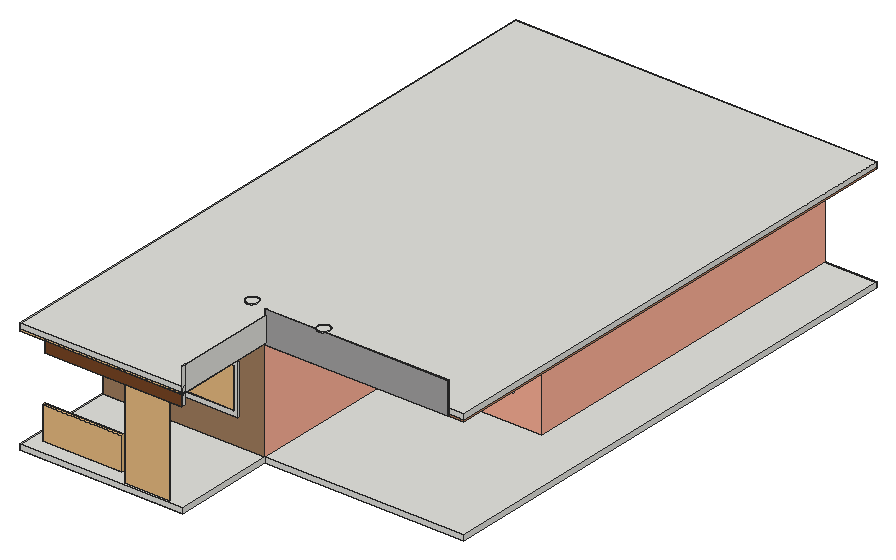
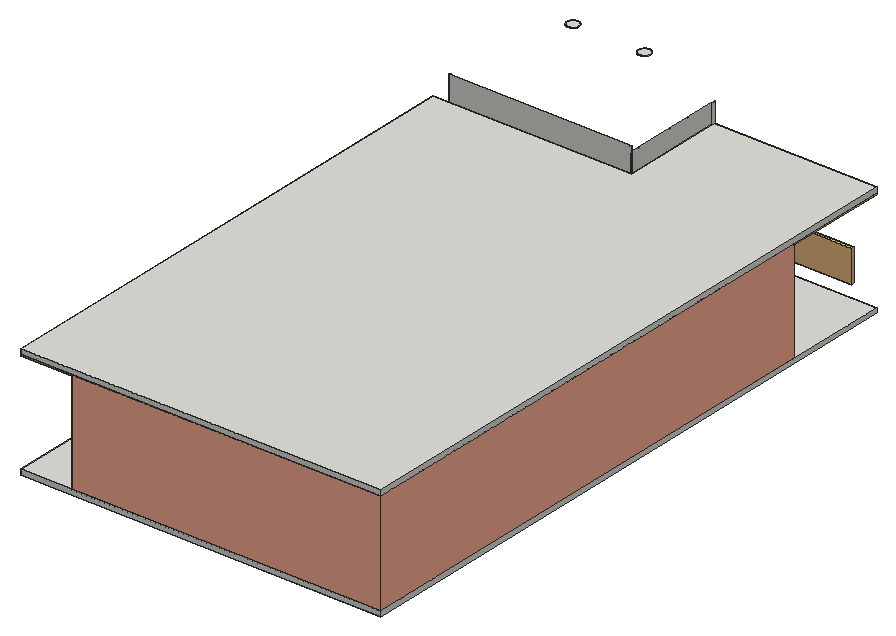
# SketchUp Ruby script. Lengths in inches.
U = 1.inch
M = Sketchup.active_model
def pt(a) = Geom::Point3d.new(a.map { |v| v * U })
def face(e, loops, mat)
  f = e.add_face(loops[0].map { |a| pt(a) })
  loops[1..].each { |l| e.add_face(l.map { |a| pt(a) }).erase! }
  f.material = f.back_material = mat if mat
  f
end
# faces: each face lists its corners as indices into pts; further lists are holes
def faces(e, pts, list, mat = nil) = list.each { |f| face(e, (f[0].is_a?(Array) ? f : [f]).map { |l| l.map { |i| pts[i] } }, mat) }
# xy, xz, yz: faces in a plane at the given z, y or x. An outline is a flat list of corners, or four numbers for a rectangle; further outlines are holes
def ring(l) = l.size == 4 ? [[l[0], l[1]], [l[2], l[1]], [l[2], l[3]], [l[0], l[3]]] : l.each_slice(2).to_a
def flat(e, list, mat, &to3) = list.each { |f| face(e, (f[0].is_a?(Array) ? f : [f]).map { |l| ring(l).map { |u, v| to3.(u, v) } }, mat) }
def xy(e, z, list, mat = nil) = flat(e, list, mat) { |x, y| [x, y, z] }
def xz(e, y, list, mat = nil) = flat(e, list, mat) { |x, z| [x, y, z] }
def yz(e, x, list, mat = nil) = flat(e, list, mat) { |y, z| [x, y, z] }
def lines(e, pts, list) = list.each { |a, b| e.add_line(pt(pts[a]), pt(pts[b])) }
# prism: a flat outline (further loops are holes) pulled along v
def prism(e, loops, v, mat = nil)
  f = face(e, loops, mat); d = Geom::Vector3d.new(v.map { |x| x * U })
  f.pushpull(f.normal.samedirection?(d) ? d.length : -d.length)
end
def box(e, o, s, mat = nil) = prism(e, [[o, [o[0] + s[0], o[1], o[2]], [o[0] + s[0], o[1] + s[1], o[2]], [o[0], o[1] + s[1], o[2]]]], [0, 0, s[2]], mat)
def at(x, y, z, deg = 0) = Geom::Transformation.translation(pt([x, y, z])) * Geom::Transformation.rotation(ORIGIN, Z_AXIS, deg.degrees)
def axes(o, x, y, z) = Geom::Transformation.new([*x, 0, *y, 0, *z, 0, *pt(o).to_a, 1])
def part(name) = M.definitions.add(name)
# library, detail: a bought-in or finely detailed component or shape, given as its bounding box
def library(name, o, s) = part(name).tap { |d| box(d.entities, o, s) }
def detail(e, o, s) = box(e.add_group.entities, o, s)
def put(e, d, t, mat = nil) = e.add_instance(d, t).tap { |i| i.material = mat if mat }
def group(e, t, mat = nil) = e.add_group.tap { |g| g.transformation = t; g.material = mat if mat }.entities
root = M.entities
M.materials.add("[Cladding Siding Tan]").color = [162, 126, 95]
M.materials.add("[Color B02]").color = [255, 178, 153]
M.materials.add("[Color B08]").color = [102, 25, 0]
M.materials.add("[Color D03]").color = [255, 216, 101]
M.materials.add("[Metal Silver]").color = [234, 233, 238]
M.materials.add("[Stone Vein Gray]").color = [166, 165, 165]
M.materials.add("[Translucent Glass Blue]").color = [100, 149, 237]
M.materials["[Translucent Glass Blue]"].alpha = 0.5
M.materials.add("[Wood Veneer 01]").color = [120, 70, 37]
M.materials.add("[Wood Veneer 02]").color = [190, 128, 91]
c1 = library("Group\#19",[0,0,0],[1024,2048,10.625])
c2 = part("modren jali")
put(c2.entities,c1,axes([1490.25,379.44,-368.22],[1,0,0],[0,0,1],[0,-1,0]))
c3 = part("Difference\#1")
xy(c3.entities,0,[[0,0,0,600,360,600,360,189,255,189,255,198,351,198,351,591,9,591,9,9,180,9,180,198,213,198,213,189,189,189,189,0]])
xy(c3.entities,36,[[81,0,153,9],[288,189,324,198]])
xy(c3.entities,78,[[24,0,48,9]])
xy(c3.entities,84,[[81,0,153,9],[213,189,255,198],[288,189,324,198]])
xy(c3.entities,102,[[24,0,48,9]])
xy(c3.entities,120,[[[0,0,189,0,189,189,360,189,360,600,0,600],[9,9,9,591,351,591,351,198,180,198,180,9]]])
xz(c3.entities,0,[[[0,0,189,120],[81,36,153,84],[24,78,48,102]]],"[Cladding Siding Tan]")
xz(c3.entities,9,[[[9,0,180,120],[81,36,153,84],[24,78,48,102]]])
xz(c3.entities,189,[[[189,0,213,0,213,84,255,84,255,0,360,0,360,120,189,120],[288,36,324,84]]])
xz(c3.entities,198,[[[180,0,180,120,351,120,351,0,255,0,255,84,213,84,213,0],[288,36,324,84]]])
xz(c3.entities,591,[[9,0,351,120]])
xz(c3.entities,600,[[0,0,360,120]])
yz(c3.entities,0,[[0,0,600,120]])
yz(c3.entities,9,[[9,0,591,120]])
yz(c3.entities,24,[[0,78,9,102]])
yz(c3.entities,48,[[0,78,9,102]])
yz(c3.entities,81,[[0,36,9,84]])
yz(c3.entities,153,[[0,36,9,84]])
yz(c3.entities,180,[[9,0,198,120]])
yz(c3.entities,189,[[0,0,189,120]])
yz(c3.entities,213,[[189,0,198,84]])
yz(c3.entities,255,[[189,0,198,84]])
yz(c3.entities,288,[[189,36,198,84]])
yz(c3.entities,324,[[189,36,198,84]])
yz(c3.entities,351,[[198,0,591,120]])
yz(c3.entities,360,[[189,0,600,120]])
c4 = library("Group\#3",[0,0,0],[47.51,11.03,86.76])
c5 = library("Group\#38",[0,0,0],[92.21,3.15,37.57])
c6 = part("Group\#9")
prism(c6.entities,[[[82.01,1,58.01],[82.01,1,0],[0,1,0],[0,1,58.01]],[[5.04,1,52.97],[5.04,1,5.04],[76.97,1,5.04],[76.97,1,52.97]]],[0,-1,0])
c7 = part("Group\#10")
prism(c7.entities,[[[42.49,0,54.49],[0,0,54.49],[0,0,0],[42.49,0,0]],[[3.28,0,51.21],[39.21,0,51.21],[39.21,0,3.28],[3.28,0,3.28]]],[0,1,0])
c8 = library("Group\#5",[0,0,0],[36,9.07,48])
c9 = library("Group\#2",[0,0,0],[72,9.07,48])
c10 = part("Group15\#2")
box(c10.entities,[1.02,2.16,1.02],[21.96,1.15,21.96])
c11 = part("Group\#7")
put(c11.entities,c10,at(0,0,0),"[Translucent Glass Blue]")
g1 = group(c11.entities,at(0,0,0),"[Metal Silver]")
xy(g1,0,[[0,0,24,9]])
xy(g1,0.83,[[0.83,4.61,23.17,8.93]])
xy(g1,1.02,[[1.02,2.16,22.98,3.3125]])
xy(g1,1.61,[[1.61,1.8,22.39,2.16]])
xy(g1,1.65,[[1.65,3.3125,22.35,3.46]])
xy(g1,22.35,[[1.65,3.3125,22.35,3.46]])
xy(g1,22.39,[[1.61,1.8,22.39,2.16]])
xy(g1,22.98,[[1.02,2.16,22.98,3.3125]])
xy(g1,23.17,[[0.83,4.61,23.17,8.93]])
xy(g1,24,[[0,0,24,9]])
xz(g1,0,[[[0,0,24,24],[0.39,0.39,23.61,23.61]]])
xz(g1,0.36,[[[0.59,0.59,23.41,23.41],[0.79,0.79,23.21,23.21]]])
xz(g1,1.8,[[[0.83,0.83,23.17,23.17],[1.61,1.61,22.39,22.39]]])
xz(g1,2.16,[[[1.02,1.02,22.98,22.98],[1.61,1.61,22.39,22.39]]])
xz(g1,3.3125,[[[1.02,1.02,22.98,22.98],[1.65,1.65,22.35,22.35]]])
xz(g1,4.61,[[[0.83,0.83,23.17,23.17],[1.5,1.5,22.5,22.5]]])
xz(g1,9.07,[[[0.04,0.04,23.96,23.96],[0.75,0.75,23.25,23.25]]])
yz(g1,0,[[0,0,9,24]])
yz(g1,0.83,[[4.61,0.83,8.93,23.17]])
yz(g1,1.02,[[2.16,1.02,3.3125,22.98]])
yz(g1,1.61,[[1.8,1.61,2.16,22.39]])
yz(g1,1.65,[[3.3125,1.65,3.46,22.35]])
yz(g1,22.35,[[3.3125,1.65,3.46,22.35]])
yz(g1,22.39,[[1.8,1.61,2.16,22.39]])
yz(g1,22.98,[[2.16,1.02,3.3125,22.98]])
yz(g1,23.17,[[4.61,0.83,8.93,23.17]])
yz(g1,24,[[0,0,9,24]])
p = [[0,9,24],[0.04,9.07,23.96],[0.04,9.07,0.04],[0,9,0],[12,9.07,0.04],[23.96,9.07,0.04],
  [24,9,0],[12,9,0],[23.96,9.07,23.96],[24,9,24],[0.59,0.36,23.41],[0.39,0,23.61],
  [0.39,0,0.39],[0.59,0.36,0.59],[12,0,0.39],[23.61,0,0.39],[23.41,0.36,0.59],[12,0.36,0.59],
  [23.61,0,23.61],[23.41,0.36,23.41],[0.75,9.07,23.25],[0.83,8.93,23.17],[0.83,8.93,0.83],[0.75,9.07,0.75],
  [12,8.93,0.83],[23.17,8.93,0.83],[23.25,9.07,0.75],[12,9.07,0.75],[23.17,8.93,23.17],[23.25,9.07,23.25],
  [0.83,1.8,23.17],[0.79,0.36,23.21],[0.79,0.36,0.79],[0.83,1.8,0.83],[12,0.36,0.79],[23.21,0.36,0.79],
  [23.17,1.8,0.83],[12,1.8,0.83],[23.21,0.36,23.21],[23.17,1.8,23.17],[1.5,4.61,22.5],[1.65,3.46,22.35],
  [1.65,3.46,1.65],[1.5,4.61,1.5],[12,3.46,1.65],[22.35,3.46,1.65],[22.5,4.61,1.5],[12,4.61,1.5],
  [22.35,3.46,22.35],[22.5,4.61,22.5]]
faces(g1,p,[[0,1,2,3],[4,5,6,7,3,2],[6,5,8,9],[10,11,12,13],[14,15,16,17,13,12],[16,15,18,19],[20,21,22,23],[24,25,26,27,23,22],
  [26,25,28,29],[30,31,32,33],[34,35,36,37,33,32],[36,35,38,39],[40,41,42,43],[44,45,46,47,43,42],[46,45,48,49],[49,48,41,40],
  [39,38,31,30],[29,28,21,20],[19,18,11,10],[9,8,1,0]])
c12 = library("Group\#14",[0,0,0],[189,120,2])
prism(root,[[[232.19,63.35,333.73],[233.86,62.6,333.73],[235.28,61.44,333.73],[236.35,59.96,333.73],[237,58.25,333.73],[237.18,56.43,333.73],[236.89,54.63,333.73],[236.14,52.96,333.73],[234.98,51.55,333.73],[233.5,50.48,333.73],[231.79,49.83,333.73],[229.98,49.64,333.73],[228.17,49.9375,333.73],[226.51,50.68,333.73],[225.09,51.84,333.73],[224.02,53.32,333.73],[223.37,55.03,333.73],[223.1875,56.85,333.73],[223.48,58.65,333.73],[224.23,60.32,333.73],[225.38,61.73,333.73],[226.86,62.8,333.73],[228.57,63.45,333.73],[230.39,63.64,333.73]]],[0,0,0.5])
prism(root,[[[315.44,63.35,333.73],[317.11,62.6,333.73],[318.53,61.44,333.73],[319.6,59.96,333.73],[320.25,58.25,333.73],[320.43,56.43,333.73],[320.14,54.63,333.73],[319.39,52.96,333.73],[318.23,51.55,333.73],[316.75,50.48,333.73],[315.04,49.83,333.73],[313.23,49.64,333.73],[311.42,49.9375,333.73],[309.76,50.68,333.73],[308.34,51.84,333.73],[307.27,53.32,333.73],[306.62,55.03,333.73],[306.4375,56.85,333.73],[306.73,58.65,333.73],[307.48,60.32,333.73],[308.63,61.73,333.73],[310.11,62.8,333.73],[311.82,63.45,333.73],[313.64,63.64,333.73]]],[0,0,0.5])
xy(root,231.87,[[30.57,5,190,6]])
xy(root,244,[[30.57,5,190,6],[190,125,403,126]])
xy(root,246,[[190,9,191,125]])
xy(root,274,[[190,9,191,125]])
xy(root,280.96,[[190,125,403,126]])
xz(root,5,[[30.57,231.87,190,244]],"[Wood Veneer 01]")
xz(root,6,[[30.57,231.87,190,244]])
xz(root,9,[[190,246,191,274]])
xz(root,125,[[190,244,403,244,403,280.96,190,280.96,190,274,191,274,191,246,190,246]],"[Stone Vein Gray]")
xz(root,126,[[190,244,403,280.96]])
yz(root,30.57,[[5,231.87,6,244]])
yz(root,190,[[5,231.87,6,231.95],[5,231.95,6,244],[6,231.95,9,244],[5,244,9,246],[125,244,126,246],
  [5,246,9,274],[5,274,9,274.64],[125,274,126,280.96]])
yz(root,191,[[9,246,125,274]])
yz(root,403,[[125,244,126,280.96]])
p = [[190,9,274.64],[190,9,280]]
lines(root,p,[[0,1]])
g2 = group(root,at(1,126,120))
prism(g2,[[[0,-120,0],[0,600,0],[420,600,0],[420,0,0],[189,0,0],[189,-120,0]]],[0,0,6])
put(root,c2,axes([246.81,26.01,147.22],[-0.0502,0,0],[0,-0.04483,0],[0,0,0.05762]))
put(root,c3,at(1,126,126),"[Color B02]")
put(root,c4,at(211.24,313.82,126))
put(root,c5,at(28.99,3.43,140.55))
put(root,c6,at(77,124.93,156.96))
put(root,c7,at(285.76,313.93,158.72))
put(root,c8,at(325,324,161.96,180))
put(root,c9,at(153.96,135.07,161.96,180),"[Color B08]")
put(root,c11,at(49,135,203.96,180))
g3 = group(root,at(190,126,244),"[Wood Veneer 02]")
xy(g3,0,[[[0,0,0,189,171,189,171,600,231,600,231,0],[138.86,155.04,140.375,155.42,141.74,156.18,142.87,157.28,143.67,158.62,144.09,160.13,144.12,161.7,143.73,163.21,142.97,164.58,141.875,165.7,140.53,166.51,139.02,166.93,137.46,166.95,135.9375,166.57,134.57,165.8,133.45,164.71,132.65,163.37,132.22,161.86,132.2,160.29,132.58,158.77,133.35,157.41,134.4375,156.28,135.78,155.48,137.29,155.06],[138.86,95.04,140.375,95.42,141.74,96.18,142.87,97.28,143.67,98.62,144.09,100.13,144.12,101.7,143.73,103.21,142.97,104.58,141.875,105.7,140.53,106.51,139.02,106.93,137.46,106.95,135.9375,106.57,134.57,105.8,133.45,104.71,132.65,103.37,132.22,101.86,132.2,100.29,132.58,98.77,133.35,97.41,134.4375,96.28,135.78,95.48,137.29,95.06],[138.86,35.04,140.375,35.42,141.74,36.18,142.87,37.28,143.67,38.62,144.09,40.13,144.12,41.7,143.73,43.21,142.97,44.58,141.875,45.7,140.53,46.51,139.02,46.93,137.46,46.95,135.9375,46.57,134.57,45.8,133.45,44.71,132.65,43.37,132.22,41.86,132.2,40.29,132.58,38.77,133.35,37.41,134.4375,36.28,135.78,35.48,137.29,35.06],[48.05,35.04,49.5625,35.42,50.93,36.18,52.05,37.28,52.86,38.62,53.28,40.13,53.3,41.7,52.92,43.21,52.15,44.58,51.0625,45.7,49.72,46.51,48.21,46.93,46.64,46.95,45.125,46.57,43.76,45.8,42.64,44.71,41.83,43.37,41.41,41.86,41.39,40.29,41.77,38.77,42.53,37.41,43.625,36.28,44.97,35.48,46.48,35.06],[48.05,95.04,49.5625,95.42,50.93,96.18,52.05,97.28,52.86,98.62,53.28,100.13,53.3,101.7,52.92,103.21,52.15,104.58,51.0625,105.7,49.72,106.51,48.21,106.93,46.64,106.95,45.125,106.57,43.76,105.8,42.64,104.71,41.83,103.37,41.41,101.86,41.39,100.29,41.77,98.77,42.53,97.41,43.625,96.28,44.97,95.48,46.48,95.06],[48.05,155.04,49.5625,155.42,50.93,156.18,52.05,157.28,52.86,158.62,53.28,160.13,53.3,161.7,52.92,163.21,52.15,164.58,51.0625,165.7,49.72,166.51,48.21,166.93,46.64,166.95,45.125,166.57,43.76,165.8,42.64,164.71,41.83,163.37,41.41,161.86,41.39,160.29,41.77,158.77,42.53,157.41,43.625,156.28,44.97,155.48,46.48,155.06]]])
xy(g3,0.5,[[48.05,35.04,46.48,35.06,44.97,35.48,43.625,36.28,42.53,37.41,41.77,38.77,41.39,40.29,41.41,41.86,41.83,43.37,42.64,44.71,43.76,45.8,45.125,46.57,46.64,46.95,48.21,46.93,49.72,46.51,51.0625,45.7,52.15,44.58,52.92,43.21,53.3,41.7,53.28,40.13,52.86,38.62,52.05,37.28,50.93,36.18,49.5625,35.42],[138.86,35.04,137.29,35.06,135.78,35.48,134.4375,36.28,133.35,37.41,132.58,38.77,132.2,40.29,132.22,41.86,132.65,43.37,133.45,44.71,134.57,45.8,135.9375,46.57,137.46,46.95,139.02,46.93,140.53,46.51,141.875,45.7,142.97,44.58,143.73,43.21,144.12,41.7,144.09,40.13,143.67,38.62,142.87,37.28,141.74,36.18,140.375,35.42],[48.05,95.04,46.48,95.06,44.97,95.48,43.625,96.28,42.53,97.41,41.77,98.77,41.39,100.29,41.41,101.86,41.83,103.37,42.64,104.71,43.76,105.8,45.125,106.57,46.64,106.95,48.21,106.93,49.72,106.51,51.0625,105.7,52.15,104.58,52.92,103.21,53.3,101.7,53.28,100.13,52.86,98.62,52.05,97.28,50.93,96.18,49.5625,95.42],[138.86,95.04,137.29,95.06,135.78,95.48,134.4375,96.28,133.35,97.41,132.58,98.77,132.2,100.29,132.22,101.86,132.65,103.37,133.45,104.71,134.57,105.8,135.9375,106.57,137.46,106.95,139.02,106.93,140.53,106.51,141.875,105.7,142.97,104.58,143.73,103.21,144.12,101.7,144.09,100.13,143.67,98.62,142.87,97.28,141.74,96.18,140.375,95.42],[48.05,155.04,46.48,155.06,44.97,155.48,43.625,156.28,42.53,157.41,41.77,158.77,41.39,160.29,41.41,161.86,41.83,163.37,42.64,164.71,43.76,165.8,45.125,166.57,46.64,166.95,48.21,166.93,49.72,166.51,51.0625,165.7,52.15,164.58,52.92,163.21,53.3,161.7,53.28,160.13,52.86,158.62,52.05,157.28,50.93,156.18,49.5625,155.42],
  [138.86,155.04,137.29,155.06,135.78,155.48,134.4375,156.28,133.35,157.41,132.58,158.77,132.2,160.29,132.22,161.86,132.65,163.37,133.45,164.71,134.57,165.8,135.9375,166.57,137.46,166.95,139.02,166.93,140.53,166.51,141.875,165.7,142.97,164.58,143.73,163.21,144.12,161.7,144.09,160.13,143.67,158.62,142.87,157.28,141.74,156.18,140.375,155.42]],"[Color D03]")
xy(g3,2,[[0,0,231,0,231,600,171,600,171,189,0,189]])
xz(g3,0,[[0,0,231,2]])
xz(g3,189,[[0,0,171,2]])
xz(g3,600,[[171,0,231,2]])
yz(g3,0,[[0,0,189,2]])
yz(g3,171,[[189,0,600,2]])
yz(g3,231,[[0,0,600,2]])
p = [[48.05,35.04,0],[46.48,35.06,0],[46.48,35.06,0.5],[48.05,35.04,0.5],[49.5625,35.42,0],[49.5625,35.42,0.5],
  [138.86,35.04,0],[137.29,35.06,0],[137.29,35.06,0.5],[138.86,35.04,0.5],[140.375,35.42,0],[140.375,35.42,0.5],
  [44.97,35.48,0],[44.97,35.48,0.5],[135.78,35.48,0],[135.78,35.48,0.5],[50.93,36.18,0],[50.93,36.18,0.5],
  [141.74,36.18,0],[141.74,36.18,0.5],[43.625,36.28,0],[43.625,36.28,0.5],[134.4375,36.28,0],[134.4375,36.28,0.5],
  [52.05,37.28,0],[52.05,37.28,0.5],[142.87,37.28,0],[142.87,37.28,0.5],[42.53,37.41,0],[42.53,37.41,0.5],
  [133.35,37.41,0],[133.35,37.41,0.5],[52.86,38.62,0],[52.86,38.62,0.5],[143.67,38.62,0],[143.67,38.62,0.5],
  [41.77,38.77,0],[41.77,38.77,0.5],[132.58,38.77,0],[132.58,38.77,0.5],[53.28,40.13,0],[53.28,40.13,0.5],
  [144.09,40.13,0],[144.09,40.13,0.5],[41.39,40.29,0],[41.39,40.29,0.5],[132.2,40.29,0],[132.2,40.29,0.5],
  [53.3,41.7,0],[53.3,41.7,0.5],[144.12,41.7,0],[144.12,41.7,0.5],[41.41,41.86,0],[41.41,41.86,0.5],
  [132.22,41.86,0],[132.22,41.86,0.5],[52.92,43.21,0],[52.92,43.21,0.5],[143.73,43.21,0],[143.73,43.21,0.5],
  [41.83,43.37,0],[41.83,43.37,0.5],[132.65,43.37,0],[132.65,43.37,0.5],[52.15,44.58,0],[52.15,44.58,0.5],
  [142.97,44.58,0],[142.97,44.58,0.5],[42.64,44.71,0],[42.64,44.71,0.5],[133.45,44.71,0],[133.45,44.71,0.5],
  [51.0625,45.7,0],[51.0625,45.7,0.5],[141.875,45.7,0],[141.875,45.7,0.5],[43.76,45.8,0],[43.76,45.8,0.5],
  [134.57,45.8,0],[134.57,45.8,0.5],[49.72,46.51,0],[49.72,46.51,0.5],[140.53,46.51,0],[140.53,46.51,0.5],
  [45.125,46.57,0],[45.125,46.57,0.5],[135.9375,46.57,0],[135.9375,46.57,0.5],[48.21,46.93,0],[48.21,46.93,0.5],
  [139.02,46.93,0],[139.02,46.93,0.5],[46.64,46.95,0],[46.64,46.95,0.5],[137.46,46.95,0],[137.46,46.95,0.5],
  [48.05,95.04,0],[46.48,95.06,0],[46.48,95.06,0.5],[48.05,95.04,0.5],[49.5625,95.42,0],[49.5625,95.42,0.5],
  [138.86,95.04,0],[137.29,95.06,0],[137.29,95.06,0.5],[138.86,95.04,0.5],[140.375,95.42,0],[140.375,95.42,0.5],
  [44.97,95.48,0],[44.97,95.48,0.5],[135.78,95.48,0],[135.78,95.48,0.5],[50.93,96.18,0],[50.93,96.18,0.5],
  [141.74,96.18,0],[141.74,96.18,0.5],[43.625,96.28,0],[43.625,96.28,0.5],[134.4375,96.28,0],[134.4375,96.28,0.5],
  [52.05,97.28,0],[52.05,97.28,0.5],[142.87,97.28,0],[142.87,97.28,0.5],[42.53,97.41,0],[42.53,97.41,0.5],
  [133.35,97.41,0],[133.35,97.41,0.5],[52.86,98.62,0],[52.86,98.62,0.5],[143.67,98.62,0],[143.67,98.62,0.5],
  [41.77,98.77,0],[41.77,98.77,0.5],[132.58,98.77,0],[132.58,98.77,0.5],[53.28,100.13,0],[53.28,100.13,0.5],
  [144.09,100.13,0],[144.09,100.13,0.5],[41.39,100.29,0],[41.39,100.29,0.5],[132.2,100.29,0],[132.2,100.29,0.5],
  [53.3,101.7,0],[53.3,101.7,0.5],[144.12,101.7,0],[144.12,101.7,0.5],[41.41,101.86,0],[41.41,101.86,0.5],
  [132.22,101.86,0],[132.22,101.86,0.5],[52.92,103.21,0],[52.92,103.21,0.5],[143.73,103.21,0],[143.73,103.21,0.5],
  [41.83,103.37,0],[41.83,103.37,0.5],[132.65,103.37,0],[132.65,103.37,0.5],[52.15,104.58,0],[52.15,104.58,0.5],
  [142.97,104.58,0],[142.97,104.58,0.5],[42.64,104.71,0],[42.64,104.71,0.5],[133.45,104.71,0],[133.45,104.71,0.5],
  [51.0625,105.7,0],[51.0625,105.7,0.5],[141.875,105.7,0],[141.875,105.7,0.5],[43.76,105.8,0],[43.76,105.8,0.5],
  [134.57,105.8,0],[134.57,105.8,0.5],[49.72,106.51,0],[49.72,106.51,0.5],[140.53,106.51,0],[140.53,106.51,0.5],
  [45.125,106.57,0],[45.125,106.57,0.5],[135.9375,106.57,0],[135.9375,106.57,0.5],[48.21,106.93,0],[48.21,106.93,0.5],
  [139.02,106.93,0],[139.02,106.93,0.5],[46.64,106.95,0],[46.64,106.95,0.5],[137.46,106.95,0],[137.46,106.95,0.5],
  [48.05,155.04,0],[46.48,155.06,0],[46.48,155.06,0.5],[48.05,155.04,0.5],[49.5625,155.42,0],[49.5625,155.42,0.5],
  [138.86,155.04,0],[137.29,155.06,0],[137.29,155.06,0.5],[138.86,155.04,0.5],[140.375,155.42,0],[140.375,155.42,0.5],
  [44.97,155.48,0],[44.97,155.48,0.5],[135.78,155.48,0],[135.78,155.48,0.5],[50.93,156.18,0],[50.93,156.18,0.5],
  [141.74,156.18,0],[141.74,156.18,0.5],[43.625,156.28,0],[43.625,156.28,0.5],[134.4375,156.28,0],[134.4375,156.28,0.5],
  [52.05,157.28,0],[52.05,157.28,0.5],[142.87,157.28,0],[142.87,157.28,0.5],[42.53,157.41,0],[42.53,157.41,0.5],
  [133.35,157.41,0],[133.35,157.41,0.5],[52.86,158.62,0],[52.86,158.62,0.5],[143.67,158.62,0],[143.67,158.62,0.5],
  [41.77,158.77,0],[41.77,158.77,0.5],[132.58,158.77,0],[132.58,158.77,0.5],[53.28,160.13,0],[53.28,160.13,0.5],
  [144.09,160.13,0],[144.09,160.13,0.5],[41.39,160.29,0],[41.39,160.29,0.5],[132.2,160.29,0],[132.2,160.29,0.5],
  [53.3,161.7,0],[53.3,161.7,0.5],[144.12,161.7,0],[144.12,161.7,0.5],[41.41,161.86,0],[41.41,161.86,0.5],
  [132.22,161.86,0],[132.22,161.86,0.5],[52.92,163.21,0],[52.92,163.21,0.5],[143.73,163.21,0],[143.73,163.21,0.5],
  [41.83,163.37,0],[41.83,163.37,0.5],[132.65,163.37,0],[132.65,163.37,0.5],[52.15,164.58,0],[52.15,164.58,0.5],
  [142.97,164.58,0],[142.97,164.58,0.5],[42.64,164.71,0],[42.64,164.71,0.5],[133.45,164.71,0],[133.45,164.71,0.5],
  [51.0625,165.7,0],[51.0625,165.7,0.5],[141.875,165.7,0],[141.875,165.7,0.5],[43.76,165.8,0],[43.76,165.8,0.5],
  [134.57,165.8,0],[134.57,165.8,0.5],[49.72,166.51,0],[49.72,166.51,0.5],[140.53,166.51,0],[140.53,166.51,0.5],
  [45.125,166.57,0],[45.125,166.57,0.5],[135.9375,166.57,0],[135.9375,166.57,0.5],[48.21,166.93,0],[48.21,166.93,0.5],
  [139.02,166.93,0],[139.02,166.93,0.5],[46.64,166.95,0],[46.64,166.95,0.5],[137.46,166.95,0],[137.46,166.95,0.5]]
faces(g3,p,[[0,1,2,3],[4,0,3,5],[6,7,8,9],[10,6,9,11],[1,12,13,2],[7,14,15,8],[16,4,5,17],[18,10,11,19],
  [12,20,21,13],[14,22,23,15],[24,16,17,25],[26,18,19,27],[20,28,29,21],[22,30,31,23],[32,24,25,33],[34,26,27,35],
  [28,36,37,29],[30,38,39,31],[40,32,33,41],[42,34,35,43],[36,44,45,37],[38,46,47,39],[48,40,41,49],[50,42,43,51],
  [44,52,53,45],[46,54,55,47],[56,48,49,57],[58,50,51,59],[52,60,61,53],[54,62,63,55],[64,56,57,65],[66,58,59,67],
  [60,68,69,61],[62,70,71,63],[72,64,65,73],[74,66,67,75],[68,76,77,69],[70,78,79,71],[80,72,73,81],[82,74,75,83],
  [76,84,85,77],[78,86,87,79],[88,80,81,89],[90,82,83,91],[84,92,93,85],[86,94,95,87],[92,88,89,93],[94,90,91,95],
  [96,97,98,99],[100,96,99,101],[102,103,104,105],[106,102,105,107],[97,108,109,98],[103,110,111,104],[112,100,101,113],[114,106,107,115],
  [108,116,117,109],[110,118,119,111],[120,112,113,121],[122,114,115,123],[116,124,125,117],[118,126,127,119],[128,120,121,129],[130,122,123,131],
  [124,132,133,125],[126,134,135,127],[136,128,129,137],[138,130,131,139],[132,140,141,133],[134,142,143,135],[144,136,137,145],[146,138,139,147],
  [140,148,149,141],[142,150,151,143],[152,144,145,153],[154,146,147,155],[148,156,157,149],[150,158,159,151],[160,152,153,161],[162,154,155,163],
  [156,164,165,157],[158,166,167,159],[168,160,161,169],[170,162,163,171],[164,172,173,165],[166,174,175,167],[176,168,169,177],[178,170,171,179],
  [172,180,181,173],[174,182,183,175],[184,176,177,185],[186,178,179,187],[180,188,189,181],[182,190,191,183],[188,184,185,189],[190,186,187,191],
  [192,193,194,195],[196,192,195,197],[198,199,200,201],[202,198,201,203],[193,204,205,194],[199,206,207,200],[208,196,197,209],[210,202,203,211],
  [204,212,213,205],[206,214,215,207],[216,208,209,217],[218,210,211,219],[212,220,221,213],[214,222,223,215],[224,216,217,225],[226,218,219,227],
  [220,228,229,221],[222,230,231,223],[232,224,225,233],[234,226,227,235],[228,236,237,229],[230,238,239,231],[240,232,233,241],[242,234,235,243],
  [236,244,245,237],[238,246,247,239],[248,240,241,249],[250,242,243,251],[244,252,253,245],[246,254,255,247],[256,248,249,257],[258,250,251,259],
  [252,260,261,253],[254,262,263,255],[264,256,257,265],[266,258,259,267],[260,268,269,261],[262,270,271,263],[272,264,265,273],[274,266,267,275],
  [268,276,277,269],[270,278,279,271],[280,272,273,281],[282,274,275,283],[276,284,285,277],[278,286,287,279],[284,280,281,285],[286,282,283,287]])
put(root,c12,at(1,6,244),"[Wood Veneer 02]")
g4 = group(root,at(1,126,246))
prism(g4,[[[0,-120,0],[0,600,0],[420,600,0],[420,0,0],[189,0,0],[189,-120,0]]],[0,0,6])
